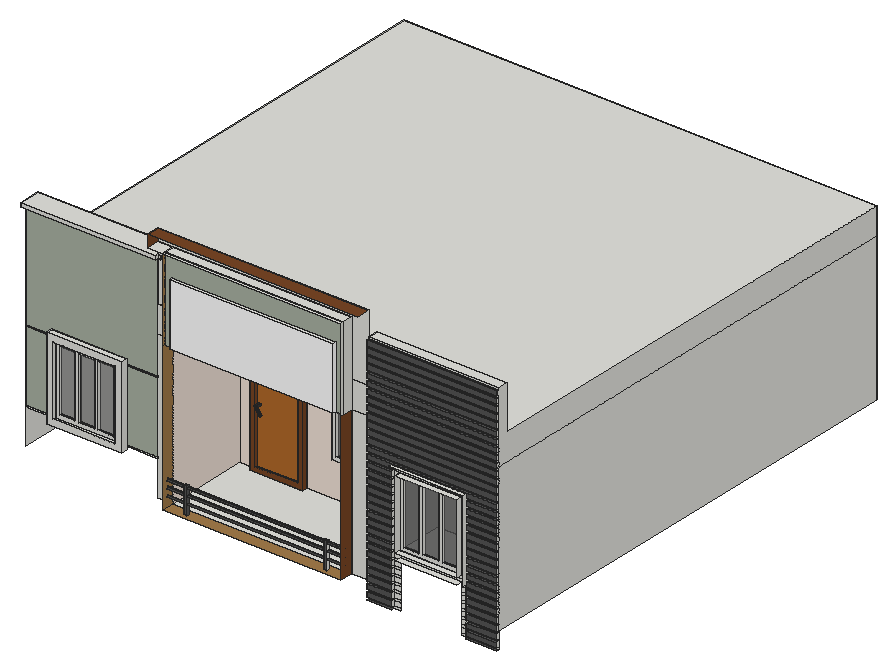
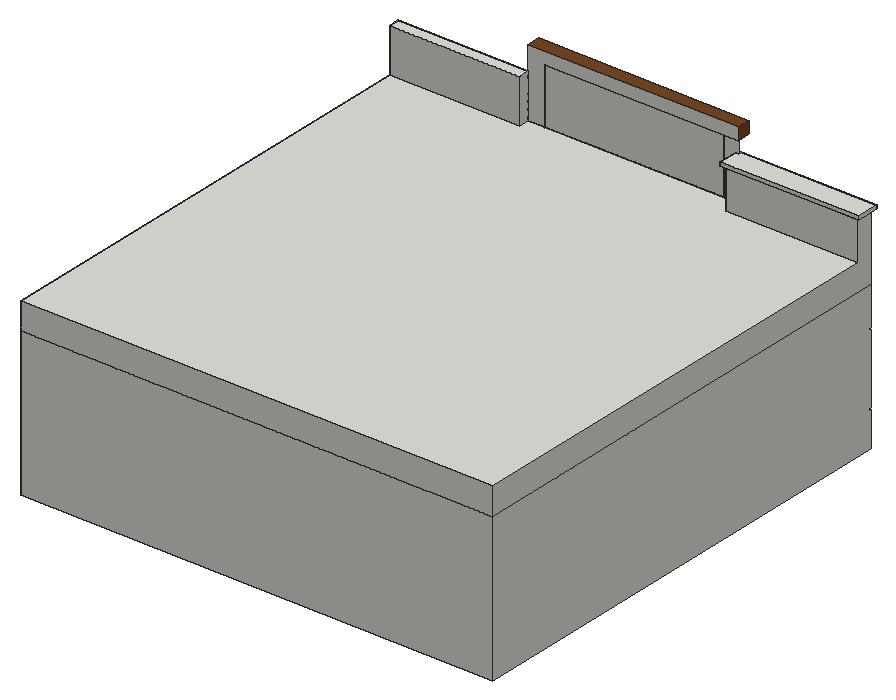
# SketchUp Ruby script. Lengths in inches.
U = 1.inch
M = Sketchup.active_model
def pt(a) = Geom::Point3d.new(a.map { |v| v * U })
def face(e, loops, mat)
  f = e.add_face(loops[0].map { |a| pt(a) })
  loops[1..].each { |l| e.add_face(l.map { |a| pt(a) }).erase! }
  f.material = f.back_material = mat if mat
  f
end
# faces: each face lists its corners as indices into pts; further lists are holes
def faces(e, pts, list, mat = nil) = list.each { |f| face(e, (f[0].is_a?(Array) ? f : [f]).map { |l| l.map { |i| pts[i] } }, mat) }
# xy, xz, yz: faces in a plane at the given z, y or x. An outline is a flat list of corners, or four numbers for a rectangle; further outlines are holes
def ring(l) = l.size == 4 ? [[l[0], l[1]], [l[2], l[1]], [l[2], l[3]], [l[0], l[3]]] : l.each_slice(2).to_a
def flat(e, list, mat, &to3) = list.each { |f| face(e, (f[0].is_a?(Array) ? f : [f]).map { |l| ring(l).map { |u, v| to3.(u, v) } }, mat) }
def xy(e, z, list, mat = nil) = flat(e, list, mat) { |x, y| [x, y, z] }
def xz(e, y, list, mat = nil) = flat(e, list, mat) { |x, z| [x, y, z] }
def yz(e, x, list, mat = nil) = flat(e, list, mat) { |y, z| [x, y, z] }
def lines(e, pts, list) = list.each { |a, b| e.add_line(pt(pts[a]), pt(pts[b])) }
# prism: a flat outline (further loops are holes) pulled along v
def prism(e, loops, v, mat = nil)
  f = face(e, loops, mat); d = Geom::Vector3d.new(v.map { |x| x * U })
  f.pushpull(f.normal.samedirection?(d) ? d.length : -d.length)
end
def box(e, o, s, mat = nil) = prism(e, [[o, [o[0] + s[0], o[1], o[2]], [o[0] + s[0], o[1] + s[1], o[2]], [o[0], o[1] + s[1], o[2]]]], [0, 0, s[2]], mat)
def at(x, y, z, deg = 0) = Geom::Transformation.translation(pt([x, y, z])) * Geom::Transformation.rotation(ORIGIN, Z_AXIS, deg.degrees)
def axes(o, x, y, z) = Geom::Transformation.new([*x, 0, *y, 0, *z, 0, *pt(o).to_a, 1])
def part(name) = M.definitions.add(name)
# library, detail: a bought-in or finely detailed component or shape, given as its bounding box
def library(name, o, s) = part(name).tap { |d| box(d.entities, o, s) }
def detail(e, o, s) = box(e.add_group.entities, o, s)
def put(e, d, t, mat = nil) = e.add_instance(d, t).tap { |i| i.material = mat if mat }
def group(e, t, mat = nil) = e.add_group.tap { |g| g.transformation = t; g.material = mat if mat }.entities
root = M.entities
M.materials.add("Generic\#1").color = [85, 85, 85]
M.materials.add("Generic\#2").color = [170, 178, 163]
M.materials.add("Generic\#3").color = [162, 123, 74]
M.materials.add("Generic\#4").color = [241, 227, 216]
M.materials.add("[Color M00]").color = [255, 255, 255]
M.materials.add("[Color M07]").color = [58, 58, 58]
M.materials.add("[Translucent Glass Gray]").color = [91, 91, 91]
M.materials["[Translucent Glass Gray]"].alpha = 0.55
M.materials.add("[Wood Bamboo]").color = [177, 105, 43]
M.materials.add("[Wood Veneer 01]").color = [120, 70, 37]
c1 = part("Group\#3")
xy(c1.entities,0,[[0,4.93,60.125,10.18]])
xy(c1.entities,5.66,[[5.66,4.93,54.46,7.18]],"[Wood Veneer 01]")
xy(c1.entities,68.44,[[8.18,1.47,8.18,7.18,9.93,7.18,9.93,2.62]],"[Color M07]")
xy(c1.entities,70.41,[[8.19,0,9.94,1.15,9.94,7.18,8.19,7.18]],"[Color M07]")
xy(c1.entities,134.78,[[5.66,4.93,54.46,7.18]])
xy(c1.entities,140.4375,[[0,4.93,60.125,10.18]],"[Wood Veneer 01]")
xz(c1.entities,4.93,[[[0,0,60.125,140.4375],[5.66,5.66,54.46,134.78]]],"[Wood Veneer 01]")
xz(c1.entities,7.18,[[[5.66,5.66,54.46,134.78],[8.18,68.44,8.19,70.41,9.94,70.41,9.93,68.44]],[8.18,68.44,8.19,70.41,9.94,70.41,9.93,68.44]],"[Wood Bamboo]")
xz(c1.entities,10.18,[[0,0,60.125,140.4375]])
yz(c1.entities,0,[[4.93,0,10.18,140.4375]],"[Wood Veneer 01]")
yz(c1.entities,5.66,[[4.93,5.66,7.18,134.78]],"[Wood Veneer 01]")
yz(c1.entities,54.46,[[4.93,5.66,7.18,134.78]],"[Wood Veneer 01]")
yz(c1.entities,60.125,[[4.93,0,10.18,140.4375]],"[Wood Veneer 01]")
p = [[8.19,0,70.41],[8.18,1.47,68.44],[14.45,1.47,61.21],[15.43,0,62.06],[15.45,2.62,62.07],[16.43,1.15,62.92],
  [9.93,2.62,68.44],[9.94,1.15,70.41],[8.19,7.18,70.41],[8.18,7.18,68.44],[9.93,7.18,68.44],[9.94,7.18,70.41],
  [8.95,0.93,69.83],[15.58,0.93,62.1875],[8.95,7.18,69.83]]
faces(c1.entities,p,[[0,1,2,3],[3,2,4,5],[1,6,4,2],[7,0,3,5],[6,7,5,4],[8,9,1,0],[10,11,7,6]],"[Color M07]")
lines(c1.entities,p,[[12,13],[14,12]])
c2 = part("Group\#2")
xy(c2.entities,0,[[0,0,74.5625,5.5]])
xy(c2.entities,4.83,[[4.83,0,23.24,2.5],[28.07,0,46.49,2.5],[51.32,0,69.73,2.5]])
xy(c2.entities,93.17,[[4.83,0,23.24,2.5],[28.07,0,46.49,2.5],[51.32,0,69.73,2.5]])
xy(c2.entities,98,[[0,0,74.5625,5.5]])
xz(c2.entities,0,[[[0,0,74.5625,98],[28.07,4.83,46.49,93.17],[51.32,4.83,69.73,93.17],[4.83,4.83,23.24,93.17]]])
xz(c2.entities,2.5,[[4.83,4.83,23.24,93.17],[28.07,4.83,46.49,93.17],[51.32,4.83,69.73,93.17]],"[Translucent Glass Gray]")
xz(c2.entities,5.5,[[0,0,74.5625,98]],"[Translucent Glass Gray]")
yz(c2.entities,0,[[0,0,5.5,98]])
yz(c2.entities,4.83,[[0,4.83,2.5,93.17]])
yz(c2.entities,23.24,[[0,4.83,2.5,93.17]])
yz(c2.entities,28.07,[[0,4.83,2.5,93.17]])
yz(c2.entities,46.49,[[0,4.83,2.5,93.17]])
yz(c2.entities,51.32,[[0,4.83,2.5,93.17]])
yz(c2.entities,69.73,[[0,4.83,2.5,93.17]])
yz(c2.entities,74.5625,[[0,0,5.5,98]])
c3 = part("Group\#1")
xy(c3.entities,0,[[0,0,70.8125,6.0625]])
xy(c3.entities,4.26,[[4.26,0,22.19,2.0625],[26.44,0,44.37,2.0625],[48.63,0,66.56,2.0625]])
xy(c3.entities,75.06,[[4.26,0,22.19,2.0625],[26.44,0,44.37,2.0625],[48.63,0,66.56,2.0625]])
xy(c3.entities,79.3125,[[0,0,70.8125,6.0625]])
xz(c3.entities,0,[[[0,0,70.8125,79.3125],[26.44,4.26,44.37,75.06],[4.26,4.26,22.19,75.06],[48.63,4.26,66.56,75.06]]])
xz(c3.entities,2.0625,[[4.26,4.26,22.19,75.06],[26.44,4.26,44.37,75.06],[48.63,4.26,66.56,75.06]],"[Translucent Glass Gray]")
xz(c3.entities,6.0625,[[0,0,70.8125,79.3125]],"[Translucent Glass Gray]")
yz(c3.entities,0,[[0,0,6.0625,79.3125]])
yz(c3.entities,4.26,[[0,4.26,2.0625,75.06]])
yz(c3.entities,22.19,[[0,4.26,2.0625,75.06]])
yz(c3.entities,26.44,[[0,4.26,2.0625,75.06]])
yz(c3.entities,44.37,[[0,4.26,2.0625,75.06]])
yz(c3.entities,48.63,[[0,4.26,2.0625,75.06]])
yz(c3.entities,66.56,[[0,4.26,2.0625,75.06]])
yz(c3.entities,70.8125,[[0,0,6.0625,79.3125]])
xy(root,776.6875,[[395.4375,28.5,423.8125,31.0625],[508.98,28.5,543.6875,31.0625]],"Generic\#1")
xy(root,779.5,[[395.4375,28.5,423.8125,31.0625],[508.98,28.5,543.6875,31.0625]],"Generic\#1")
xy(root,785,[[395.4375,28.5,423.8125,31.0625],[508.98,28.5,543.6875,31.0625]],"Generic\#1")
xy(root,787.8125,[[395.4375,28.5,423.8125,31.0625],[508.98,28.5,543.6875,31.0625]],"Generic\#1")
xy(root,793.3125,[[395.4375,28.5,423.8125,31.0625],[508.98,28.5,543.6875,31.0625]],"Generic\#1")
xy(root,795.5,[[191.29,21.49,195.1,24.24],[351.46,21.49,355.27,24.24],[171.6875,31.0625,171.6875,127,187.38,127,187.38,189.8125,247.51,189.8125,247.51,127,375.6875,127,375.6875,31.0625]])
xy(root,795.5,[[[171.6875,15.8125,375.6875,31.0625],[191.29,21.49,195.1,24.24],[351.46,21.49,355.27,24.24]]],"Generic\#3")
xy(root,796.125,[[395.4375,28.5,423.8125,31.0625],[508.98,28.5,543.6875,31.0625]],"Generic\#1")
xy(root,801.625,[[395.4375,28.5,423.8125,31.0625],[508.98,28.5,543.6875,31.0625]],"Generic\#1")
xy(root,804.4375,[[395.4375,28.5,423.8125,31.0625],[508.98,28.5,543.6875,31.0625]],"Generic\#1")
xy(root,806.32,[[171.6875,21.82,375.6875,23.63]],"Generic\#1")
xy(root,807.94,[[171.6875,21.82,375.6875,23.63]],"Generic\#1")
xy(root,809.9375,[[395.4375,28.5,423.8125,31.0625],[508.98,28.5,543.6875,31.0625]],"Generic\#1")
xy(root,812.75,[[395.4375,28.5,423.8125,31.0625],[508.98,28.5,543.6875,31.0625]],"Generic\#1")
xy(root,814.75,[[171.6875,21.82,375.6875,23.63]],"Generic\#1")
xy(root,816.38,[[171.6875,21.82,375.6875,23.63]],"Generic\#1")
xy(root,818.25,[[395.4375,28.5,423.8125,31.0625],[508.98,28.5,543.6875,31.0625]],"Generic\#1")
xy(root,821.0625,[[395.4375,28.5,423.8125,31.0625],[508.98,28.5,543.6875,31.0625]],"Generic\#1")
xy(root,823.19,[[171.6875,21.82,375.6875,23.63]],"Generic\#1")
xy(root,824.82,[[351.46,23.63,355.27,24.24]])
xy(root,824.82,[[171.6875,21.82,351.46,23.63],[355.27,21.82,375.6875,23.63]],"Generic\#1")
xy(root,825.63,[[191.29,21.49,195.1,24.24],[351.46,21.49,355.27,24.24]],"Generic\#1")
xy(root,826.5625,[[395.4375,28.5,423.8125,31.0625],[508.98,28.5,543.6875,31.0625]],"Generic\#1")
xy(root,829.375,[[395.4375,28.5,423.8125,31.0625],[508.98,28.5,543.6875,31.0625]],"Generic\#1")
xy(root,831.53,[[33.1875,24.0625,118.35,31.0625],[431.91,24.0625,501.98,31.0625]])
xy(root,834.72,[[275.98,127,350.54,182.9375]])
xy(root,834.875,[[395.4375,28.5,423.8125,31.0625],[508.98,28.5,543.6875,31.0625]],"Generic\#1")
xy(root,835.5,[[3.6875,31.0625,33.1875,32.9375],[118.35,31.0625,154.5,32.9375]])
xy(root,837.5,[[3.6875,31.0625,33.1875,32.9375],[118.35,31.0625,154.5,32.9375]])
xy(root,837.6875,[[395.4375,28.5,423.8125,31.0625],[508.98,28.5,543.6875,31.0625]],"Generic\#1")
xy(root,838.7,[[40.36,24.0625,111.18,31.0625],[430.99,24.0625,501.8,31.0625],[40.36,31.0625,111.18,85.4375],[430.99,31.0625,501.8,85.4375]])
xy(root,843.1875,[[395.4375,28.5,423.8125,31.0625],[508.98,28.5,543.6875,31.0625]],"Generic\#1")
xy(root,846,[[395.4375,28.5,423.8125,31.0625],[508.98,28.5,543.6875,31.0625]],"Generic\#1")
xy(root,851.5,[[395.4375,28.5,423.8125,31.0625],[508.98,28.5,543.6875,31.0625]],"Generic\#1")
xy(root,854.3125,[[395.4375,28.5,423.8125,31.0625],[508.98,28.5,543.6875,31.0625]],"Generic\#1")
xy(root,859.8125,[[395.4375,28.5,423.8125,31.0625],[508.98,28.5,543.6875,31.0625]],"Generic\#1")
xy(root,862.625,[[395.4375,28.5,423.8125,31.0625],[508.98,28.5,543.6875,31.0625]],"Generic\#1")
xy(root,868.125,[[395.4375,28.5,423.8125,31.0625],[508.98,28.5,543.6875,31.0625]],"Generic\#1")
xy(root,870.9375,[[395.4375,28.5,423.8125,31.0625],[508.98,28.5,543.6875,31.0625]],"Generic\#1")
xy(root,876.4375,[[395.4375,28.5,423.8125,31.0625],[508.98,28.5,543.6875,31.0625]],"Generic\#1")
xy(root,879.25,[[395.4375,28.5,423.8125,31.0625],[508.98,28.5,543.6875,31.0625]],"Generic\#1")
xy(root,884.75,[[395.4375,28.5,423.8125,31.0625],[508.98,28.5,543.6875,31.0625]],"Generic\#1")
xy(root,887.5625,[[395.4375,28.5,423.8125,31.0625],[508.98,28.5,543.6875,31.0625]],"Generic\#1")
xy(root,893.0625,[[395.4375,28.5,423.8125,31.0625],[508.98,28.5,543.6875,31.0625]],"Generic\#1")
xy(root,895.875,[[395.4375,28.5,423.8125,31.0625],[508.98,28.5,543.6875,31.0625]],"Generic\#1")
xy(root,901.375,[[395.4375,28.5,423.8125,31.0625],[508.98,28.5,543.6875,31.0625]],"Generic\#1")
xy(root,904.1875,[[395.4375,28.5,423.8125,31.0625],[508.98,28.5,543.6875,31.0625]],"Generic\#1")
xy(root,909.6875,[[395.4375,28.5,423.8125,31.0625],[508.98,28.5,543.6875,31.0625]],"Generic\#1")
xy(root,912.5,[[395.4375,28.5,423.8125,31.0625],[508.98,28.5,543.6875,31.0625]],"Generic\#1")
xy(root,917.9375,[[3.6875,31.0625,33.1875,32.9375],[118.35,31.0625,154.5,32.9375]])
xy(root,918,[[395.4375,28.5,423.8125,31.0625],[508.98,28.5,543.6875,31.0625]],"Generic\#1")
xy(root,918.02,[[40.36,24.0625,111.18,31.0625],[430.99,24.0625,501.8,31.0625],[40.36,31.0625,111.18,85.4375],[430.99,31.0625,501.8,85.4375]])
xy(root,919.9375,[[3.6875,31.0625,33.1875,32.9375],[118.35,31.0625,154.5,32.9375]])
xy(root,920.8125,[[395.4375,28.5,423.8125,31.0625],[508.98,28.5,543.6875,31.0625]],"Generic\#1")
xy(root,925.19,[[33.1875,24.0625,118.35,31.0625],[423.8125,24.0625,508.98,28.5],[423.8125,28.5,508.98,31.0625]])
xy(root,926.3125,[[395.4375,28.5,543.6875,31.0625]],"Generic\#1")
xy(root,929.125,[[395.4375,28.5,543.6875,31.0625]],"Generic\#1")
xy(root,932.72,[[275.98,127,350.54,182.9375]])
xy(root,934.625,[[395.4375,28.5,543.6875,31.0625]],"Generic\#1")
xy(root,935.9375,[[187.38,127,247.51,189.8125]])
xy(root,937.4375,[[395.4375,28.5,543.6875,31.0625]],"Generic\#1")
xy(root,942.9375,[[395.4375,28.5,543.6875,31.0625]],"Generic\#1")
xy(root,945.75,[[395.4375,28.5,543.6875,31.0625]],"Generic\#1")
xy(root,951.25,[[395.4375,28.5,543.6875,31.0625]],"Generic\#1")
xy(root,954.0625,[[395.4375,28.5,543.6875,31.0625]],"Generic\#1")
xy(root,959.5625,[[395.4375,28.5,543.6875,31.0625]],"Generic\#1")
xy(root,962.375,[[395.4375,28.5,543.6875,31.0625]],"Generic\#1")
xy(root,963.5,[[180.44,15.0625,366.94,19],[171.6875,19,375.6875,31.0625],[171.6875,31.0625,375.6875,127]])
xy(root,967.875,[[395.4375,28.5,543.6875,31.0625]],"Generic\#1")
xy(root,970.6875,[[395.4375,28.5,543.6875,31.0625]],"Generic\#1")
xy(root,976.1875,[[395.4375,28.5,543.6875,31.0625]],"Generic\#1")
xy(root,979,[[395.4375,28.5,543.6875,31.0625]],"Generic\#1")
xy(root,984.5,[[395.4375,28.5,543.6875,31.0625]],"Generic\#1")
xy(root,987.3125,[[395.4375,28.5,543.6875,31.0625]],"Generic\#1")
xy(root,992.8125,[[395.4375,28.5,543.6875,31.0625]],"Generic\#1")
xy(root,994.375,[[154.5,31.0625,395.4375,31.0625,395.4375,43.25,543.6875,43.25,543.6875,571.0625,3.6875,571.0625,3.6875,49.0625,154.5,49.0625]])
xy(root,995.625,[[395.4375,28.5,543.6875,31.0625]],"Generic\#1")
xy(root,1001.125,[[395.4375,28.5,543.6875,31.0625]],"Generic\#1")
xy(root,1003.9375,[[395.4375,28.5,543.6875,31.0625]],"Generic\#1")
xy(root,1009.4375,[[395.4375,28.5,543.6875,31.0625]],"Generic\#1")
xy(root,1012.25,[[395.4375,28.5,543.6875,31.0625]],"Generic\#1")
xy(root,1017.75,[[395.4375,28.5,543.6875,31.0625]],"Generic\#1")
xy(root,1020.5625,[[395.4375,28.5,543.6875,31.0625]],"Generic\#1")
xy(root,1026.0625,[[395.4375,28.5,543.6875,31.0625]],"Generic\#1")
xy(root,1028.875,[[395.4375,28.5,543.6875,31.0625]],"Generic\#1")
xy(root,1034.375,[[395.4375,28.5,543.6875,31.0625]],"Generic\#1")
xy(root,1034.53,[[180.44,15.0625,366.94,19]])
xy(root,1037.1875,[[395.4375,30.75,543.6875,31.0625]])
xy(root,1037.1875,[[395.4375,28.1875,543.6875,30.75]],"Generic\#1")
xy(root,1040.6875,[[0,27.375,154.5,31.0625],[0,31.0625,3.6875,52.75],[3.6875,31.0625,154.5,49.0625],[154.5,31.0625,158.1875,52.75],[3.6875,49.0625,154.5,52.75]])
xy(root,1042.6875,[[395.4375,30.75,543.6875,31.0625]])
xy(root,1042.6875,[[395.4375,28.1875,543.6875,30.75]],"Generic\#1")
xy(root,1044.8125,[[0,27.375,154.5,27.375,154.5,31.0625,158.1875,31.0625,158.1875,52.75,0,52.75],[395.4375,31.0625,543.6875,43.25]])
xy(root,1058.1875,[[154.5,15.8125,171.6875,31.0625],[171.6875,15.8125,375.6875,19],[171.6875,19,375.6875,31.0625]])
xy(root,1071.875,[[154.5,15.8125,395.4375,31.0625]],"[Wood Veneer 01]")
xz(root,15.0625,[[180.44,963.5,366.94,1034.53]],"[Color M00]")
xz(root,19,[[171.6875,963.5,180.44,963.5,180.44,1034.53,366.94,1034.53,366.94,963.5,375.6875,963.5,375.6875,1058.1875,171.6875,1058.1875]],"Generic\#2")
xz(root,21.49,[[191.29,795.5,195.1,825.63],[351.46,795.5,355.27,825.63]],"Generic\#1")
xz(root,21.82,[[171.6875,806.32,375.6875,807.94],[171.6875,814.75,375.6875,816.38],[171.6875,823.19,375.6875,824.82]],"Generic\#1")
xz(root,23.63,[[171.6875,806.32,375.6875,807.94],[171.6875,814.75,375.6875,816.38],[171.6875,823.19,375.6875,824.82]])
xz(root,24.0625,[[[33.1875,831.53,118.35,925.19],[40.36,838.7,111.18,918.02]]])
xz(root,24.24,[[191.29,795.5,195.1,825.63],[351.46,795.5,355.27,824.82],[351.46,824.82,355.27,825.63]])
xz(root,27.375,[[0,1040.6875,154.5,1044.8125]])
xz(root,28.1875,[[395.4375,1037.1875,543.6875,1042.6875]],"Generic\#1")
xz(root,28.5,[[395.4375,779.5,423.8125,785],[508.98,779.5,543.6875,785],[395.4375,787.8125,423.8125,793.3125],[508.98,787.8125,543.6875,793.3125],[395.4375,796.125,423.8125,801.625],
  [508.98,796.125,543.6875,801.625],[395.4375,804.4375,423.8125,809.9375],[508.98,804.4375,543.6875,809.9375],[395.4375,812.75,423.8125,818.25],[508.98,812.75,543.6875,818.25],
  [395.4375,821.0625,423.8125,826.5625],[508.98,821.0625,543.6875,826.5625],[395.4375,829.375,423.8125,834.875],[508.98,829.375,543.6875,834.875],[395.4375,837.6875,423.8125,843.1875],
  [508.98,837.6875,543.6875,843.1875],[395.4375,846,423.8125,851.5],[508.98,846,543.6875,851.5],[395.4375,854.3125,423.8125,859.8125],[508.98,854.3125,543.6875,859.8125],
  [395.4375,862.625,423.8125,868.125],[508.98,862.625,543.6875,868.125],[395.4375,870.9375,423.8125,876.4375],[508.98,870.9375,543.6875,876.4375],[395.4375,879.25,423.8125,884.75],
  [508.98,879.25,543.6875,884.75],[395.4375,887.5625,423.8125,893.0625],[508.98,887.5625,543.6875,893.0625],[395.4375,895.875,423.8125,901.375],[508.98,895.875,543.6875,901.375],
  [395.4375,904.1875,423.8125,909.6875],[508.98,904.1875,543.6875,909.6875],[395.4375,912.5,423.8125,918],[508.98,912.5,543.6875,918],[395.4375,920.8125,423.8125,920.8125,423.8125,925.19,508.98,925.19,508.98,920.8125,543.6875,920.8125,543.6875,926.3125,395.4375,926.3125],
  [395.4375,929.125,543.6875,934.625],[395.4375,937.4375,543.6875,942.9375],[395.4375,945.75,543.6875,951.25],[395.4375,954.0625,543.6875,959.5625],[395.4375,962.375,543.6875,967.875],
  [395.4375,970.6875,543.6875,976.1875],[395.4375,979,543.6875,984.5],[395.4375,987.3125,543.6875,992.8125],[395.4375,995.625,543.6875,1001.125],[395.4375,1003.9375,543.6875,1009.4375],
  [395.4375,1012.25,543.6875,1017.75],[395.4375,1020.5625,543.6875,1026.0625],[395.4375,1028.875,543.6875,1034.375]],"Generic\#1")
xz(root,30.75,[[395.4375,1037.1875,543.6875,1042.6875]])
xz(root,31.0625,[[395.4375,776.6875,423.8125,779.5],[423.8125,776.6875,431.91,779.5],[501.98,776.6875,508.98,779.5],[508.98,776.6875,543.6875,779.5],[395.4375,779.5,423.8125,785],
  [423.8125,779.5,431.91,785],[501.98,779.5,508.98,785],[508.98,779.5,543.6875,785],[395.4375,785,423.8125,787.8125],[423.8125,785,431.91,787.8125],
  [501.98,785,508.98,787.8125],[508.98,785,543.6875,787.8125],[395.4375,787.8125,423.8125,793.3125],[423.8125,787.8125,431.91,793.3125],[501.98,787.8125,508.98,793.3125],
  [508.98,787.8125,543.6875,793.3125],[395.4375,793.3125,423.8125,796.125],[423.8125,793.3125,431.91,796.125],[501.98,793.3125,508.98,796.125],[508.98,793.3125,543.6875,796.125],
  [154.5,795.5,171.6875,963.5],[375.6875,795.5,395.4375,963.5],[395.4375,796.125,423.8125,801.625],[423.8125,796.125,431.91,801.625],[501.98,796.125,508.98,801.625],
  [508.98,796.125,543.6875,801.625],[395.4375,801.625,423.8125,804.4375],[423.8125,801.625,431.91,804.4375],[501.98,801.625,508.98,804.4375],[508.98,801.625,543.6875,804.4375],
  [395.4375,804.4375,423.8125,809.9375],[423.8125,804.4375,431.91,809.9375],[501.98,804.4375,508.98,809.9375],[508.98,804.4375,543.6875,809.9375],[395.4375,809.9375,423.8125,812.75],
  [423.8125,809.9375,431.91,812.75],[501.98,809.9375,508.98,812.75],[508.98,809.9375,543.6875,812.75],[395.4375,812.75,423.8125,818.25],[423.8125,812.75,431.91,818.25],
  [501.98,812.75,508.98,818.25],[508.98,812.75,543.6875,818.25],[395.4375,818.25,423.8125,821.0625],[423.8125,818.25,431.91,821.0625],[501.98,818.25,508.98,821.0625],
  [508.98,818.25,543.6875,821.0625],[395.4375,821.0625,423.8125,826.5625],[423.8125,821.0625,431.91,826.5625],[501.98,821.0625,508.98,826.5625],[508.98,821.0625,543.6875,826.5625],
  [395.4375,826.5625,423.8125,829.375],[423.8125,826.5625,431.91,829.375],[501.98,826.5625,508.98,829.375],[508.98,826.5625,543.6875,829.375],[395.4375,829.375,423.8125,834.875],
  [423.8125,829.375,431.91,829.375,431.91,831.53,508.98,831.53,508.98,834.875,423.8125,834.875],[501.98,829.375,508.98,831.53],[508.98,829.375,543.6875,834.875],[33.1875,831.53,118.35,835.5],[395.4375,834.875,423.8125,837.6875],
  [423.8125,834.875,508.98,837.6875],[508.98,834.875,543.6875,837.6875],[33.1875,835.5,118.35,837.5],[33.1875,837.5,118.35,837.5,118.35,917.9375,111.18,917.9375,111.18,838.7,40.36,838.7,40.36,917.9375,33.1875,917.9375],[395.4375,837.6875,423.8125,843.1875],
  [423.8125,837.6875,508.98,837.6875,508.98,843.1875,501.8,843.1875,501.8,838.7,430.99,838.7,430.99,843.1875,423.8125,843.1875],[508.98,837.6875,543.6875,843.1875],[40.36,838.7,111.18,917.9375],[395.4375,843.1875,423.8125,846],[423.8125,843.1875,430.99,846],
  [501.8,843.1875,508.98,846],[508.98,843.1875,543.6875,846],[395.4375,846,423.8125,851.5],[423.8125,846,430.99,851.5],[501.8,846,508.98,851.5],
  [508.98,846,543.6875,851.5],[395.4375,851.5,423.8125,854.3125],[423.8125,851.5,430.99,854.3125],[501.8,851.5,508.98,854.3125],[508.98,851.5,543.6875,854.3125],
  [395.4375,854.3125,423.8125,859.8125],[423.8125,854.3125,430.99,859.8125],[501.8,854.3125,508.98,859.8125],[508.98,854.3125,543.6875,859.8125],[395.4375,859.8125,423.8125,862.625],
  [423.8125,859.8125,430.99,862.625],[501.8,859.8125,508.98,862.625],[508.98,859.8125,543.6875,862.625],[395.4375,862.625,423.8125,868.125],[423.8125,862.625,430.99,868.125],
  [501.8,862.625,508.98,868.125],[508.98,862.625,543.6875,868.125],[395.4375,868.125,423.8125,870.9375],[423.8125,868.125,430.99,870.9375],[501.8,868.125,508.98,870.9375],
  [508.98,868.125,543.6875,870.9375],[395.4375,870.9375,423.8125,876.4375],[423.8125,870.9375,430.99,876.4375],[501.8,870.9375,508.98,876.4375],[508.98,870.9375,543.6875,876.4375],
  [395.4375,876.4375,423.8125,879.25],[423.8125,876.4375,430.99,879.25],[501.8,876.4375,508.98,879.25],[508.98,876.4375,543.6875,879.25],[395.4375,879.25,423.8125,884.75],
  [423.8125,879.25,430.99,884.75],[501.8,879.25,508.98,884.75],[508.98,879.25,543.6875,884.75],[395.4375,884.75,423.8125,887.5625],[423.8125,884.75,430.99,887.5625],
  [501.8,884.75,508.98,887.5625],[508.98,884.75,543.6875,887.5625],[395.4375,887.5625,423.8125,893.0625],[423.8125,887.5625,430.99,893.0625],[501.8,887.5625,508.98,893.0625],
  [508.98,887.5625,543.6875,893.0625],[395.4375,893.0625,423.8125,895.875],[423.8125,893.0625,430.99,895.875],[501.8,893.0625,508.98,895.875],[508.98,893.0625,543.6875,895.875],
  [395.4375,895.875,423.8125,901.375],[423.8125,895.875,430.99,901.375],[501.8,895.875,508.98,901.375],[508.98,895.875,543.6875,901.375],[395.4375,901.375,423.8125,904.1875],
  [423.8125,901.375,430.99,904.1875],[501.8,901.375,508.98,904.1875],[508.98,901.375,543.6875,904.1875],[395.4375,904.1875,423.8125,909.6875],[423.8125,904.1875,430.99,909.6875],
  [501.8,904.1875,508.98,909.6875],[508.98,904.1875,543.6875,909.6875],[395.4375,909.6875,423.8125,912.5],[423.8125,909.6875,430.99,912.5],[501.8,909.6875,508.98,912.5],
  [508.98,909.6875,543.6875,912.5],[395.4375,912.5,423.8125,918],[423.8125,912.5,430.99,918],[501.8,912.5,508.98,918],[508.98,912.5,543.6875,918],
  [33.1875,917.9375,40.36,917.9375,40.36,918.02,111.18,918.02,111.18,917.9375,118.35,917.9375,118.35,919.9375,33.1875,919.9375],[40.36,917.9375,111.18,918.02],[395.4375,918,423.8125,920.8125],[423.8125,918,423.8125,920.8125,508.98,920.8125,508.98,918,501.8,918,501.8,918.02,430.99,918.02,430.99,918],[508.98,918,543.6875,920.8125],
  [33.1875,919.9375,118.35,925.19],[395.4375,920.8125,395.4375,926.3125,543.6875,926.3125,543.6875,920.8125,508.98,920.8125,508.98,925.19,423.8125,925.19,423.8125,920.8125],[423.8125,920.8125,508.98,925.19],[395.4375,926.3125,543.6875,929.125],[395.4375,929.125,543.6875,934.625],
  [395.4375,934.625,543.6875,937.4375],[395.4375,937.4375,543.6875,942.9375],[395.4375,942.9375,543.6875,945.75],[395.4375,945.75,543.6875,951.25],[395.4375,951.25,543.6875,954.0625],
  [395.4375,954.0625,543.6875,959.5625],[395.4375,959.5625,543.6875,962.375],[395.4375,962.375,543.6875,967.875],[154.5,963.5,171.6875,994.375],[171.6875,963.5,375.6875,994.375],
  [375.6875,963.5,395.4375,994.375],[395.4375,967.875,543.6875,970.6875],[395.4375,970.6875,543.6875,976.1875],[395.4375,976.1875,543.6875,979],[395.4375,979,543.6875,984.5],
  [395.4375,984.5,543.6875,987.3125],[395.4375,987.3125,543.6875,992.8125],[395.4375,992.8125,543.6875,995.625],[154.5,994.375,154.5,1040.6875,158.1875,1040.6875,158.1875,1044.8125,154.5,1044.8125,154.5,1058.1875,171.6875,1058.1875,171.6875,994.375],[375.6875,994.375,375.6875,1058.1875,154.5,1058.1875,154.5,1071.875,395.4375,1071.875,395.4375,994.375],
  [171.6875,994.375,375.6875,1058.1875],[395.4375,995.625,543.6875,1001.125],[395.4375,1001.125,543.6875,1003.9375],[395.4375,1003.9375,543.6875,1009.4375],[395.4375,1009.4375,543.6875,1012.25],
  [395.4375,1012.25,543.6875,1017.75],[395.4375,1017.75,543.6875,1020.5625],[395.4375,1020.5625,543.6875,1026.0625],[395.4375,1026.0625,543.6875,1028.875],[395.4375,1028.875,543.6875,1034.375],
  [395.4375,1034.375,543.6875,1037.1875],[154.5,1040.6875,158.1875,1044.8125],[395.4375,1042.6875,543.6875,1044.8125]])
xz(root,31.0625,[[33.1875,835.5,33.1875,917.9375,3.6875,917.9375,3.6875,837.5,154.5,837.5,154.5,917.9375,118.35,917.9375,118.35,835.5],[3.6875,919.9375,33.1875,919.9375,33.1875,925.19,118.35,925.19,118.35,919.9375,154.5,919.9375,154.5,1040.6875,3.6875,1040.6875]],"Generic\#2")
xz(root,32.9375,[[3.6875,835.5,33.1875,837.5],[118.35,835.5,154.5,837.5],[3.6875,917.9375,33.1875,919.9375],[118.35,917.9375,154.5,919.9375]],"Generic\#1")
xz(root,43.25,[[395.4375,994.375,543.6875,1044.8125]])
xz(root,49.0625,[[3.6875,994.375,154.5,1040.6875]])
xz(root,52.75,[[0,1040.6875,158.1875,1044.8125]])
xz(root,85.4375,[[40.36,838.7,111.18,918.02],[430.99,838.7,501.8,918.02]])
xz(root,127,[[[171.6875,795.5,187.38,795.5,187.38,935.9375,247.51,935.9375,247.51,795.5,375.6875,795.5,375.6875,963.5,171.6875,963.5],[275.98,834.72,350.54,932.72]]],"Generic\#4")
xz(root,182.9375,[[275.98,834.72,350.54,932.72]])
xz(root,189.8125,[[187.38,795.5,247.51,935.9375]])
xz(root,571.0625,[[3.6875,795.5,543.6875,963.5],[3.6875,963.5,543.6875,994.375]])
yz(root,0,[[27.375,1040.6875,52.75,1044.8125]])
yz(root,3.6875,[[31.0625,795.5,31.0625,835.5,32.9375,835.5,32.9375,837.5,31.0625,837.5,31.0625,917.9375,32.9375,917.9375,32.9375,919.9375,31.0625,919.9375,31.0625,963.5,571.0625,963.5,571.0625,795.5],[31.0625,963.5,31.0625,1040.6875,49.0625,1040.6875,49.0625,994.375,571.0625,994.375,571.0625,963.5]])
yz(root,33.1875,[[24.0625,831.53,31.0625,925.19],[31.0625,835.5,32.9375,837.5],[31.0625,917.9375,32.9375,919.9375]])
yz(root,40.36,[[24.0625,838.7,31.0625,918.02],[31.0625,838.7,85.4375,918.02]])
yz(root,111.18,[[24.0625,838.7,31.0625,918.02],[31.0625,838.7,85.4375,918.02]])
yz(root,118.35,[[24.0625,831.53,31.0625,925.19],[31.0625,835.5,32.9375,837.5],[31.0625,917.9375,32.9375,919.9375]])
yz(root,154.5,[[31.0625,835.5,32.9375,837.5],[31.0625,917.9375,32.9375,919.9375],[31.0625,994.375,49.0625,1040.6875],[27.375,1040.6875,31.0625,1044.8125]])
yz(root,154.5,[[15.8125,1058.1875,31.0625,1071.875]],"[Wood Veneer 01]")
yz(root,158.1875,[[31.0625,1040.6875,52.75,1044.8125]])
yz(root,171.6875,[[21.82,806.32,23.63,807.94],[21.82,814.75,23.63,816.38],[21.82,823.19,23.63,824.82],[19,963.5,31.0625,1058.1875]])
yz(root,171.6875,[[[15.8125,795.5,31.0625,963.5],[21.82,806.32,23.63,807.94],[21.82,814.75,23.63,816.38],[21.82,823.19,23.63,824.82]],[15.8125,963.5,19,1058.1875]],"Generic\#3")
yz(root,171.6875,[[31.0625,795.5,127,963.5]],"Generic\#4")
yz(root,180.44,[[15.0625,963.5,19,1034.53]])
yz(root,187.38,[[127,795.5,189.8125,935.9375]])
yz(root,191.29,[[21.49,795.5,24.24,825.63]],"Generic\#1")
yz(root,195.1,[[21.49,795.5,24.24,825.63]],"Generic\#1")
yz(root,247.51,[[127,795.5,189.8125,935.9375]])
yz(root,275.98,[[127,834.72,182.9375,932.72]])
yz(root,350.54,[[127,834.72,182.9375,932.72]])
yz(root,351.46,[[21.49,824.82,21.82,825.63],[21.82,824.82,23.63,825.63],[23.63,824.82,24.24,825.63]])
yz(root,351.46,[[21.49,795.5,24.24,824.82]],"Generic\#1")
yz(root,355.27,[[21.49,795.5,24.24,824.82],[21.49,824.82,21.82,825.63],[21.82,824.82,23.63,825.63],[23.63,824.82,24.24,825.63]])
yz(root,366.94,[[15.0625,963.5,19,1034.53]],"[Color M00]")
yz(root,375.6875,[[15.8125,963.5,19,1058.1875],[19,963.5,31.0625,1058.1875]])
yz(root,375.6875,[[31.0625,795.5,127,963.5]],"Generic\#4")
yz(root,375.6875,[[[15.8125,795.5,31.0625,963.5],[21.82,806.32,23.63,807.94],[21.82,814.75,23.63,816.38],[21.82,823.19,23.63,824.82]]],"[Wood Veneer 01]")
yz(root,395.4375,[[28.5,779.5,31.0625,785],[28.5,787.8125,31.0625,793.3125],[28.5,796.125,31.0625,801.625],[28.5,804.4375,31.0625,809.9375],[28.5,812.75,31.0625,818.25],
  [28.5,821.0625,31.0625,826.5625],[28.5,829.375,31.0625,834.875],[28.5,837.6875,31.0625,843.1875],[28.5,846,31.0625,851.5],[28.5,854.3125,31.0625,859.8125],
  [28.5,862.625,31.0625,868.125],[28.5,870.9375,31.0625,876.4375],[28.5,879.25,31.0625,884.75],[28.5,887.5625,31.0625,893.0625],[28.5,895.875,31.0625,901.375],
  [28.5,904.1875,31.0625,909.6875],[28.5,912.5,31.0625,918],[28.5,920.8125,31.0625,926.3125],[28.5,929.125,31.0625,934.625],[28.5,937.4375,31.0625,942.9375],
  [28.5,945.75,31.0625,951.25],[28.5,954.0625,31.0625,959.5625],[28.5,962.375,31.0625,963.5],[28.5,963.5,31.0625,967.875],[28.5,970.6875,31.0625,976.1875],
  [28.5,979,31.0625,984.5],[28.5,987.3125,31.0625,992.8125],[31.0625,994.375,43.25,1044.8125],[28.5,995.625,31.0625,1001.125],[28.5,1003.9375,31.0625,1009.4375],
  [28.5,1012.25,31.0625,1017.75],[28.5,1020.5625,31.0625,1026.0625],[28.5,1028.875,31.0625,1034.375],[28.1875,1037.1875,30.75,1042.6875],[30.75,1037.1875,31.0625,1042.6875]])
yz(root,423.8125,[[28.5,779.5,31.0625,785],[28.5,787.8125,31.0625,793.3125],[28.5,796.125,31.0625,801.625],[28.5,804.4375,31.0625,809.9375],[28.5,812.75,31.0625,818.25],
  [28.5,821.0625,31.0625,826.5625],[28.5,829.375,31.0625,834.875],[28.5,837.6875,31.0625,843.1875],[28.5,846,31.0625,851.5],[28.5,854.3125,31.0625,859.8125],
  [28.5,862.625,31.0625,868.125],[28.5,870.9375,31.0625,876.4375],[28.5,879.25,31.0625,884.75],[28.5,887.5625,31.0625,893.0625],[28.5,895.875,31.0625,901.375],
  [28.5,904.1875,31.0625,909.6875],[28.5,912.5,31.0625,918],[28.5,920.8125,31.0625,925.19]])
yz(root,430.99,[[24.0625,838.7,31.0625,918.02],[31.0625,838.7,85.4375,918.02]])
yz(root,501.8,[[24.0625,838.7,31.0625,918.02],[31.0625,838.7,85.4375,918.02]])
yz(root,508.98,[[28.5,779.5,31.0625,785],[28.5,787.8125,31.0625,793.3125],[28.5,796.125,31.0625,801.625],[28.5,804.4375,31.0625,809.9375],[28.5,812.75,31.0625,818.25],
  [28.5,821.0625,31.0625,826.5625],[28.5,829.375,31.0625,831.53],[24.0625,831.53,28.5,831.53,28.5,834.875,31.0625,834.875,31.0625,837.6875,28.5,837.6875,28.5,843.1875,31.0625,843.1875,31.0625,846,28.5,846,28.5,851.5,31.0625,851.5,31.0625,854.3125,28.5,854.3125,28.5,859.8125,31.0625,859.8125,31.0625,862.625,28.5,862.625,28.5,868.125,31.0625,868.125,31.0625,870.9375,28.5,870.9375,28.5,876.4375,31.0625,876.4375,31.0625,879.25,28.5,879.25,28.5,884.75,31.0625,884.75,31.0625,887.5625,28.5,887.5625,28.5,893.0625,31.0625,893.0625,31.0625,895.875,28.5,895.875,28.5,901.375,31.0625,901.375,31.0625,904.1875,28.5,904.1875,28.5,909.6875,31.0625,909.6875,31.0625,912.5,28.5,912.5,28.5,918,31.0625,918,31.0625,920.8125,28.5,920.8125,28.5,925.19,24.0625,925.19],[28.5,831.53,31.0625,834.875],[28.5,837.6875,31.0625,843.1875],
  [28.5,846,31.0625,851.5],[28.5,854.3125,31.0625,859.8125],[28.5,862.625,31.0625,868.125],[28.5,870.9375,31.0625,876.4375],[28.5,879.25,31.0625,884.75],
  [28.5,887.5625,31.0625,893.0625],[28.5,895.875,31.0625,901.375],[28.5,904.1875,31.0625,909.6875],[28.5,912.5,31.0625,918],[28.5,920.8125,31.0625,925.19]])
yz(root,543.6875,[[28.5,779.5,31.0625,785],[28.5,787.8125,31.0625,793.3125],[31.0625,795.5,571.0625,963.5],[28.5,796.125,31.0625,801.625],[28.5,804.4375,31.0625,809.9375],
  [28.5,812.75,31.0625,818.25],[28.5,821.0625,31.0625,826.5625],[28.5,829.375,31.0625,834.875],[28.5,837.6875,31.0625,843.1875],[28.5,846,31.0625,851.5],
  [28.5,854.3125,31.0625,859.8125],[28.5,862.625,31.0625,868.125],[28.5,870.9375,31.0625,876.4375],[28.5,879.25,31.0625,884.75],[28.5,887.5625,31.0625,893.0625],
  [28.5,895.875,31.0625,901.375],[28.5,904.1875,31.0625,909.6875],[28.5,912.5,31.0625,918],[28.5,920.8125,31.0625,926.3125],[28.5,929.125,31.0625,934.625],
  [28.5,937.4375,31.0625,942.9375],[28.5,945.75,31.0625,951.25],[28.5,954.0625,31.0625,959.5625],[28.5,962.375,31.0625,963.5],[28.5,963.5,31.0625,967.875],
  [31.0625,963.5,571.0625,963.5,571.0625,994.375,43.25,994.375,43.25,1044.8125,31.0625,1044.8125,31.0625,1042.6875,30.75,1042.6875,30.75,1037.1875,31.0625,1037.1875],[28.5,970.6875,31.0625,976.1875],[28.5,979,31.0625,984.5],[28.5,987.3125,31.0625,992.8125],[28.5,995.625,31.0625,1001.125],
  [28.5,1003.9375,31.0625,1009.4375],[28.5,1012.25,31.0625,1017.75],[28.5,1020.5625,31.0625,1026.0625],[28.5,1028.875,31.0625,1034.375],[28.1875,1037.1875,30.75,1042.6875]])
p = [[171.6875,22.58,807.28],[193.23,22.58,807.28],[171.6875,22.58,815.85],[193.23,22.58,815.85],[171.6875,22.58,824.41],[193.23,22.58,824.41],
  [353.55,22.58,824.41],[375.6875,22.58,824.41],[353.55,22.58,815.85],[353.55,22.58,807.28],[375.6875,22.58,807.28],[375.6875,22.58,815.85],
  [353.55,22.58,795.5],[193.23,22.58,795.5],[430.99,31.0625,918],[501.8,31.0625,918]]
lines(root,p,[[0,1],[2,3],[4,5],[6,7],[6,8],[9,10],[8,11],[9,12],[8,9],[5,3],[1,13],[3,1],
  [1,9],[3,8],[5,6],[14,15]])
put(root,c1,at(187.38,116.82,795.5))
put(root,c2,at(275.98,127,834.72))
put(root,c3,at(40.36,27.5625,838.7))
put(root,c3,at(430.99,31.0625,838.7))
